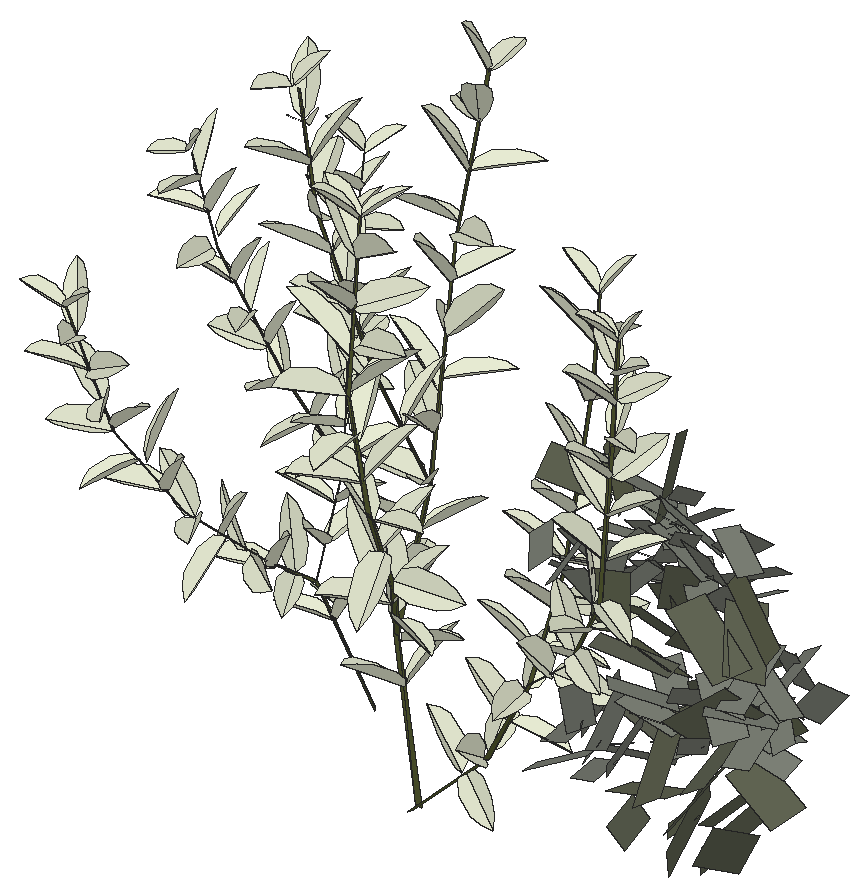
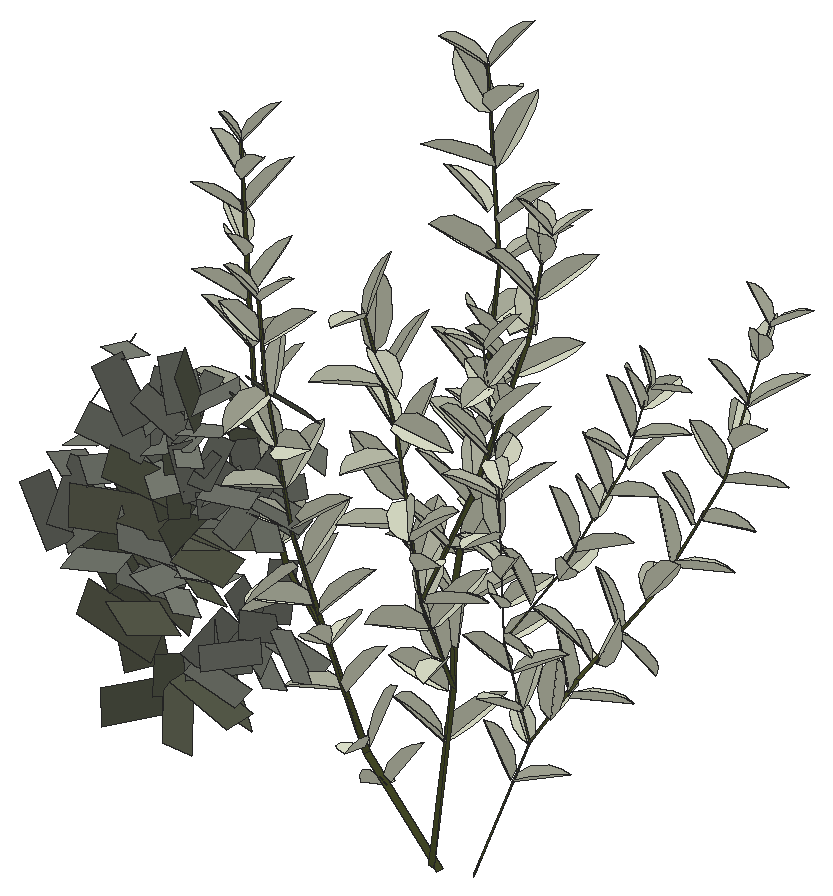
# SketchUp Ruby script. Lengths in inches.
U = 1.inch
M = Sketchup.active_model
def pt(a) = Geom::Point3d.new(a.map { |v| v * U })
def face(e, loops, mat)
  f = e.add_face(loops[0].map { |a| pt(a) })
  loops[1..].each { |l| e.add_face(l.map { |a| pt(a) }).erase! }
  f.material = f.back_material = mat if mat
  f
end
# faces: each face lists its corners as indices into pts; further lists are holes
def faces(e, pts, list, mat = nil) = list.each { |f| face(e, (f[0].is_a?(Array) ? f : [f]).map { |l| l.map { |i| pts[i] } }, mat) }
# xy, xz, yz: faces in a plane at the given z, y or x. An outline is a flat list of corners, or four numbers for a rectangle; further outlines are holes
def ring(l) = l.size == 4 ? [[l[0], l[1]], [l[2], l[1]], [l[2], l[3]], [l[0], l[3]]] : l.each_slice(2).to_a
def flat(e, list, mat, &to3) = list.each { |f| face(e, (f[0].is_a?(Array) ? f : [f]).map { |l| ring(l).map { |u, v| to3.(u, v) } }, mat) }
def xy(e, z, list, mat = nil) = flat(e, list, mat) { |x, y| [x, y, z] }
def xz(e, y, list, mat = nil) = flat(e, list, mat) { |x, z| [x, y, z] }
def yz(e, x, list, mat = nil) = flat(e, list, mat) { |y, z| [x, y, z] }
def lines(e, pts, list) = list.each { |a, b| e.add_line(pt(pts[a]), pt(pts[b])) }
# prism: a flat outline (further loops are holes) pulled along v
def prism(e, loops, v, mat = nil)
  f = face(e, loops, mat); d = Geom::Vector3d.new(v.map { |x| x * U })
  f.pushpull(f.normal.samedirection?(d) ? d.length : -d.length)
end
def box(e, o, s, mat = nil) = prism(e, [[o, [o[0] + s[0], o[1], o[2]], [o[0] + s[0], o[1] + s[1], o[2]], [o[0], o[1] + s[1], o[2]]]], [0, 0, s[2]], mat)
def at(x, y, z, deg = 0) = Geom::Transformation.translation(pt([x, y, z])) * Geom::Transformation.rotation(ORIGIN, Z_AXIS, deg.degrees)
def axes(o, x, y, z) = Geom::Transformation.new([*x, 0, *y, 0, *z, 0, *pt(o).to_a, 1])
def part(name) = M.definitions.add(name)
# library, detail: a bought-in or finely detailed component or shape, given as its bounding box
def library(name, o, s) = part(name).tap { |d| box(d.entities, o, s) }
def detail(e, o, s) = box(e.add_group.entities, o, s)
def put(e, d, t, mat = nil) = e.add_instance(d, t).tap { |i| i.material = mat if mat }
def group(e, t, mat = nil) = e.add_group.tap { |g| g.transformation = t; g.material = mat if mat }.entities
root = M.entities
M.materials.add("0ad16as01f6asdLeafVar1sfd015as60f1as6").color = [231, 235, 211]
M.materials.add("asdfasdf0165f6asdLeafVar1sfd015as60f1as6").color = [231, 235, 211]
M.materials.add("dw_stemssadfasdfa0sdf1s01d6w1").color = [90, 97, 50]
M.materials.add("viburnumblaasdfas0df1w06d").color = [98, 102, 84]
M.materials.add("viburnumbladsadfasdfad0w122").color = [125, 129, 119]
c1 = part("vdw_leaf\#1")
p = [[0,0,0],[-2.77,1.61,2.32],[-4.3125,6.1,4.5],[-3.97,13.49,6.09],[-2.47,18.57,6.3],[-0.2,22.73,5.75],
  [2.54,19.66,6.85],[4.3,15.93,7.09],[5.03,7.6,5.43],[3.32,1.76,2.74]]
faces(c1.entities,p,[[0,1,2,3,4,5],[0,5,6,7,8,9]],"0ad16as01f6asdLeafVar1sfd015as60f1as6")
c2 = part("dw_branch_3\#2")
p = [[-10.06,-1.6,62.9],[-0.2,1.54,-0.01],[-10.43,1.54,62.72],[0.18,-1.6,0.17],[-23.75,-21.66,88.91],[-25.7,-20.3,89.55],
  [13.4,11.62,104.56],[13.33,13.52,104.47],[-49.25,-41.87,130.3125],[-50.33,-40.21,130.71],[-4.97,21.13,143.98],[35.61,27.99,178.64],
  [-5.09,23.64,143.96],[35.32,29.14,178.46],[-67.7,-55.38,181.06],[-68.34,-54.45,181.62],[-22.8125,33.9,200.59],[-22.94,35.79,200.41],
  [56.61,36.78,229.75],[56.29,38.09,229.57],[-70.63,-67.46,248.85],[-70.72,-66.33,249.5],[-25.05,43.32,240.75],[-24.98,44.26,240.57]]
faces(c2.entities,p,[[0,1,2],[0,3,1],[4,2,5],[4,0,2],[6,0,2],[6,2,7],[8,4,5],[8,5,9],
  [10,6,7],[11,6,7],[10,7,12],[11,7,13],[14,8,9],[14,9,15],[16,10,12],[16,12,17],
  [18,11,13],[18,13,19],[20,14,15],[20,15,21],[22,16,17],[22,17,23]],"dw_stemssadfasdfa0sdf1s01d6w1")
c3 = part("dw_branch3\#2")
put(c3.entities,c1,axes([-70.33,-63.58,233.32],[-1.00752,0.412,0.78596],[-0.24851,-1.22189,0.32195],[0.83141,0.09817,1.01433]))
put(c3.entities,c1,axes([-66.93,-54.91,182.82],[-0.84976,-0.98359,0.33619],[0.99572,-0.74889,0.32577],[-0.05223,0.46521,1.22907]))
put(c3.entities,c1,axes([-46.12,-39.49,126.35],[1.23843,0.5364,0.23552],[-0.56438,0.94474,0.81599],[0.15707,-0.83465,1.07498]))
put(c3.entities,c1,axes([13.0625,13.13,104.77],[-1.01271,0.69982,-0.26884],[-0.74268,-0.99813,0.19939],[-0.10222,0.31872,1.21473]))
put(c3.entities,c1,axes([-18.87,30.42,186.42],[0.36309,1.06515,-0.56675],[-1.14134,0.49515,0.19939],[0.39128,0.45593,1.10754]))
put(c3.entities,c1,axes([-3.2,4.15,75.77],[-1.04153,0.55414,0.44243],[-0.23365,-1.01045,0.71554],[0.6695,0.50943,0.93801]))
put(c3.entities,c1,axes([23.2,19.41,136.3],[-0.65687,-1.11295,-0.05714],[1.05857,-0.61429,-0.20411],[0.15163,-0.1536,1.24868]))
put(c3.entities,c1,axes([-25.57,35.48,201.32],[-0.64726,0.62827,0.87973],[-0.71635,-1.0172,0.19939],[0.80962,-0.39773,0.87973]))
put(c3.entities,c1,axes([-36.37,-32.14,110.35],[-0.80747,1.09962,0.12544],[-0.83333,-0.50188,-0.96467],[-0.72833,-0.64487,0.96467]))
put(c3.entities,c1,axes([-9.89,26.72,156.79],[0.45529,1.02969,0.56572],[-1.16919,0.33753,0.32662],[0.11537,-0.64297,1.07744]))
put(c3.entities,c1,axes([-26.57,46.1,241.0625],[0.00015,0.80921,0.22536],[-0.83985,0.00446,-0.01542],[-0.01605,-0.22532,0.80906]))
put(c3.entities,c1,axes([-9.2,-2.58,61.06],[-1.10001,-0.40312,0.39014],[0.40883,-1.1116,0.00411],[0.35732,0.13566,1.14763]))
put(c3.entities,c1,axes([-69.91,-63.11,233.93],[1.36249,-0.1432,0],[0.13201,1.25603,0.5309],[-0.05549,-0.52799,1.26295]))
put(c3.entities,c1,axes([32.2,25.46,166.13],[0.06878,-1.29051,-0.05714],[1.22165,0.07415,-0.20411],[0.2113,-0.04403,1.24868]))
put(c3.entities,c1,axes([-5.68,-0.66,44.43],[-0.48448,-1.12287,0.17078],[0.98138,-0.33653,0.57135],[-0.48308,0.36756,1.04626]))
put(c3.entities,c1,axes([43.45,32.81,198.64],[0.5408,1.19584,0.14106],[-0.94242,0.32409,0.86557],[0.74952,-0.45533,0.98656]))
put(c3.entities,c1,axes([12.52,14.14,104.98],[1.02694,0.54888,0.41092],[-0.53566,1.05407,-0.06927],[-0.38969,-0.12321,1.13846]))
put(c3.entities,c1,axes([44.55,32.375,198.73],[-0.65687,-1.11295,-0.05714],[1.05857,-0.61429,-0.20411],[0.15163,-0.1536,1.24868]))
put(c3.entities,c1,axes([-5.67,21.17,141.44],[-1.10726,0.43603,-0.32953],[-0.49537,-1.03435,0.29588],[-0.17521,0.40597,1.12589]))
put(c3.entities,c1,axes([55.69,37.84,229.48],[0.18984,0.96334,0.18958],[-0.71996,0.0053,0.69399],[0.66755,-0.26823,0.69457]))
put(c3.entities,c1,axes([-21.52,36.85,205.2],[0.72606,-0.98817,0.14519],[0.94364,0.7084,0.10251],[-0.16885,0.05176,1.19664]))
put(c3.entities,c1,axes([-68.51,-56.35,196.07],[1.16319,0.72381,0],[-0.66725,1.0723,0.5309],[0.28049,-0.45075,1.26295]))
put(c3.entities,c2,at(0.01,-0.09,-0.02),"dw_stemssadfasdfa0sdf1s01d6w1")
put(c3.entities,c1,axes([-2.49,5.18,75.91],[0.78614,-0.90346,-0.30078],[0.86953,0.79562,-0.11715],[0.28546,-0.14014,1.16705]))
put(c3.entities,c1,axes([-23.125,-16.22,82.25],[0.32175,1.32576,0.12544],[-1.33153,0.31835,0.05068],[0.01989,-0.13382,1.3633]))
put(c3.entities,c1,axes([-23.75,41.99,230.3],[0.85958,-0.87451,0.14519],[0.66531,0.75721,0.62192],[-0.54076,-0.36226,1.01955]))
put(c3.entities,c1,axes([27.07,22.48,149.34],[0.92952,-0.64745,-0.62467],[0.50188,1.074,-0.36637],[0.71693,0.02135,1.04468]))
put(c3.entities,c1,axes([17.66,16.25,119.93],[-0.91649,0.83891,-0.3601],[-0.87434,-0.77966,0.40896],[0.0492,0.54447,1.14321]))
put(c3.entities,c1,axes([-68.37,-54.54,181.63],[0.32047,1.28399,0.35434],[-1.33153,0.31835,0.05068],[-0.03484,-0.35624,1.32241]))
put(c3.entities,c1,axes([-28.98,-27.1,96.48],[-0.8814,-0.35966,-0.98523],[0.75246,-1.11336,-0.26672],[-0.73065,-0.71272,0.91382]))
put(c3.entities,c1,axes([-15.23,28.43,172.72],[-1.21149,0.11898,0.32517],[-0.09739,-1.25259,0.09551],[0.33228,0.0667,1.21356]))
put(c3.entities,c1,axes([-17.5625,31.23,186.85],[-0.49275,-1.12287,0.14519],[0.95014,-0.33653,0.62192],[-0.53717,0.36756,1.01955]))
put(c3.entities,c1,axes([26.7,21.22,149.39],[-1.00104,0.22334,0.83093],[0.36894,-1.0402,0.72406],[0.77731,0.78134,0.72643]))
put(c3.entities,c1,axes([-31.125,-24.87,97.38],[0.75482,-0.86936,0.69068],[-0.00159,0.80023,1.00899],[-1.08766,-0.58016,0.45842]))
put(c3.entities,c1,axes([-71.21,-66.73,248.67],[0.25207,0.96771,0],[-0.8921,0.23237,0.38752],[0.375,-0.09768,0.92186]))
put(c3.entities,c1,axes([-24.11,41.05,229.55],[-1.11612,0.51924,-0.26884],[-0.56394,-1.10897,0.19939],[-0.15444,0.29694,1.21473]))
put(c3.entities,c1,axes([6.75,8.37,91.63],[-0.33418,-1.12287,0.39014],[1.13558,-0.33653,0.00411],[0.10478,0.36756,1.14763]))
put(c3.entities,c1,axes([-26,45.89,241.63],[-0.26986,-0.70824,-0.32129],[0.56818,-0.39091,0.38449],[-0.49365,-0.09775,0.63011]))
put(c3.entities,c1,axes([3.74,17.32,124.35],[0.22441,1.22913,-0.16274],[-1.07812,0.11178,-0.64246],[-0.61228,0.25367,1.07162]))
put(c3.entities,c1,axes([-5.44,22.27,140.88],[1.2203,0.00475,0.31374],[-0.097,1.20386,0.35905],[-0.29841,-0.37189,1.1663]))
put(c3.entities,c1,axes([-13.79,29.35,173.31],[0.83169,-0.90108,0.14519],[0.68877,0.73594,0.62192],[-0.55187,-0.34509,1.01955]))
put(c3.entities,c1,axes([-16.92,-7.26,72.98],[1.30647,0.30378,-0.27886],[0.07026,0.74892,1.14503],[0.40633,-1.10623,0.69861]))
put(c3.entities,c1,axes([4.8,17.55,125.22],[-0.25598,-1.17842,0.26559],[1.01553,-0.08455,0.60363],[-0.56975,0.35087,1.00767]))
put(c3.entities,c1,axes([5.3125,8.35,91.45],[0.00638,1.22913,-0.27714],[-1.16413,0.11178,0.46895],[0.48205,0.25367,1.13617]))
put(c3.entities,c1,axes([38.12,30.57,183.07],[1.12534,0.26182,-0.63833],[-0.46674,1.18829,-0.33545],[0.5081,0.51169,1.10563]))
put(c3.entities,c1,axes([-70.41,-60.38,214.47],[-0.41425,1.30587,0],[-1.20383,-0.38188,0.5309],[0.50605,0.16053,1.26295]))
put(c3.entities,c1,axes([37.03,28.75,180.67],[-1.12533,0.00102,-0.63799],[-0.00113,-1.2408,0],[-0.62497,0.00057,1.10237]))
put(c3.entities,c1,axes([30.71,25.35,165.96],[-0.1364,1.29314,0.22715],[-1.08768,-0.23921,0.70862],[0.73536,-0.11394,1.09026]))
put(c3.entities,c1,axes([-38.05,-30.84,110.67],[-0.31533,-1.27379,-0.2839],[1.018,-0.40311,0.67794],[-0.74394,-0.05723,1.08307]))
put(c3.entities,c1,axes([50.11,34.45,213.36],[-1.05669,0.74401,-0.05714],[-0.616,-0.82138,0.69675],[0.37221,0.60904,1.04705]))
put(c3.entities,c1,axes([-65.32,-58.78,200.07],[-1.14597,-0.19668,-0.6713],[0.21784,-1.26924,0],[-0.64812,-0.11124,1.139]))
put(c3.entities,c1,axes([-53.2,-43.37,143.59],[-0.72817,-1.09167,-0.2839],[0.82127,-0.72411,0.67794],[-0.71934,0.19815,1.08307]))
put(c3.entities,c1,axes([-61.1,-50.25,163.67],[-0.52887,1.19686,-0.30066],[-1.10762,-0.57104,-0.32484],[-0.42634,0.12264,1.23812]))
put(c3.entities,c1,axes([-54.12,-42.96,142.67],[0.32175,1.32576,0.12544],[-1.33153,0.31835,0.05068],[0.01989,-0.13382,1.3633]))
put(c3.entities,c1,axes([22.03,20.08,132.3],[1.17066,0.5058,-0.34078],[-0.35758,1.16671,0.50333],[0.49407,-0.35407,1.17172]))
put(c3.entities,c1,axes([-8.59,26.04,158.21],[-0.49275,-1.12287,0.14519],[0.95014,-0.33653,0.62192],[-0.53717,0.36756,1.01955]))
put(c3.entities,c1,axes([49.92,34.03,213.7],[1.24742,-0.35176,0.25024],[0.42127,1.159,-0.4708],[-0.09426,0.52477,1.20753]))
put(c3.entities,c1,axes([-70.34,-67.02,249.05],[-0.57048,-0.79684,0],[0.73827,-0.52855,0.24329],[-0.20203,0.14464,0.92729]))
put(c3.entities,c1,axes([56.04,36.81,228.63],[0.33451,-0.90845,-0.15237],[0.87636,0.33365,-0.06538],[0.11487,-0.11636,0.94597]))
put(c3.entities,c1,axes([-69.93,-60.58,214.88],[-0.45293,-0.99272,-0.78227],[1.14635,-0.58199,0.07483],[-0.40282,-0.65636,1.06615]))
put(c3.entities,c1,axes([-16.77,-8.59,72.7],[-1.22785,0.11509,0.53076],[-0.24879,-1.22495,-0.30991],[0.46742,-0.38989,1.16587]))
put(c3.entities,c1,axes([18.29,17.18,119.24],[1.19981,-0.45946,0.3029],[0.40159,1.22775,0.27158],[-0.37626,-0.1547,1.25575]))
put(c3.entities,c1,axes([-6.73,-0.68,43.74],[0.05346,1.22913,-0.27201],[-1.22696,0.11178,0.26396],[0.28163,0.25367,1.20164]))
put(c3.entities,c1,axes([-58.57,-48.42,160.98],[0.43385,-1.23789,0.39533],[1.04879,0.57965,0.66404],[-0.76727,0.09236,1.13122]))
put(c3.entities,c1,axes([-23.4,38.49,215.38],[0.06762,1.22913,-0.26884],[-1.23909,0.11178,0.19939],[0.21835,0.25367,1.21473]))
put(c3.entities,c1,axes([-22.21,-16.62,83.17],[-0.72817,-1.09167,-0.2839],[0.82127,-0.72411,0.67794],[-0.71934,0.19815,1.08307]))
put(c3.entities,c1,axes([-45.7,-40.77,126.53],[-1.33715,-0.0713,-0.0976],[0.07167,-1.28508,-0.04314],[-0.09306,-0.0492,1.31098]))
put(c3.entities,c1,axes([-22.39,38.51,216.12],[-0.49275,-1.12287,0.14519],[0.95014,-0.33653,0.62192],[-0.53717,0.36756,1.01955]))
c4 = part("Component\#315")
p = [[0.25,0,0],[2.05,0.01,0.35],[1.81,4.2,1.66],[0,4.19,1.3125]]
faces(c4.entities,p,[[0,1,2,3]],"viburnumbladsadfasdfad0w122")
c5 = part("viburnumblad2")
put(c5.entities,c4,axes([-19.23,-4.49,-32.18],[83.35428,0,0],[0,79.38502,0],[0,0,83.35428]))
c6 = part("vdw_leaf\#2")
p = [[0,0,0],[-2.77,1.61,2.32],[-4.3125,6.1,4.5],[-3.97,13.49,6.09],[-2.47,18.57,6.3],[-0.2,22.73,5.75],
  [2.54,19.66,6.85],[4.3,15.93,7.09],[5.03,7.6,5.43],[3.32,1.76,2.74]]
faces(c6.entities,p,[[0,1,2,3,4,5],[0,5,6,7,8,9]],"asdfasdf0165f6asdLeafVar1sfd015as60f1as6")
c7 = part("dg_branch_1\#2")
p = [[46.12,1.57,35.62],[46,5.42,35.41],[0.14,1.79,0.05],[0.26,-2.0625,0.27],[74.05,2.99,75.8],[74.11,5.28,75.58],
  [103.46,0.47,94.74],[104.03,2.92,94.84],[81.14,16.92,120.46],[81.2,18.78,120.24],[130.47,-5.6875,130.27],[130.58,-3.66,129.85],
  [80.82,34.4375,191.22],[80.64,35.93,190.9],[148.49,-14.56,203.24],[148.9,-12.8125,203.11],[81.08,37.95,226.93],[81.4,39.1,227.03],
  [157.45,-18.19,250.77],[157.7,-17.01,250.41]]
faces(c7.entities,p,[[0,1,2,3],[4,0,1],[4,1,5],[6,4,5],[6,5,7],[8,4,5],[8,5,9],[10,6,7],
  [10,7,11],[12,8,9],[12,9,13],[14,10,11],[14,11,15],[16,12,13],[16,13,17],[18,14,15],
  [18,15,19]],"dw_stemssadfasdfa0sdf1s01d6w1")
c8 = part("vdw_branch1\#3")
put(c8.entities,c6,axes([120.69,-2.42,117.31],[1.12221,-0.24063,-0.65809],[0.19207,1.24776,-0.12871],[0.65778,0.01392,1.11658]))
put(c8.entities,c6,axes([81,38.9,226.05],[0.7888,-0.58155,0],[0.48308,0.65523,0.47],[-0.28484,-0.38635,0.83138]))
put(c8.entities,c6,axes([78.08,12.69,106.05],[-1.43826,-0.02353,-0.03177],[0.0088,-1.31777,0.57755],[-0.03854,0.57714,1.31741]))
put(c8.entities,c6,axes([130.18,-4.73,130.41],[-0.38031,-1.29044,-0.11242],[1.20662,-0.31032,-0.51987],[0.47109,-0.24694,1.24081]))
put(c8.entities,c6,axes([157.08,-17.89,249.93],[-0.91355,0.40674,0],[-0.37496,-0.84216,0.38752],[0.15762,0.35401,0.92186]))
put(c8.entities,c6,axes([90.64,3.03,86.49],[0.32514,-0.85045,-0.99675],[0.69523,0.98247,-0.61148],[1.11061,-0.36604,0.67459]))
put(c8.entities,c6,axes([80.15,28.42,160.95],[-0.16039,0.95636,-1.06292],[-1.41646,0.03966,0.24943],[0.19509,1.07422,0.93709]))
put(c8.entities,c6,axes([126.74,-5.45,129.22],[-0.59819,0.96152,-0.6841],[-0.85772,0.12575,0.92675],[0.75427,0.88089,0.57856]))
put(c8.entities,c6,axes([133.22,-6.12,150.66],[-0.93823,0.76985,0.59124],[-0.47726,-1.08188,0.65135],[0.84525,0.24366,1.02405]))
put(c8.entities,c6,axes([80.43,22.89,141.32],[-1.42571,-0.19312,0.01373],[0.18338,-1.31425,0.5561],[-0.0621,0.5528,1.32692]))
put(c8.entities,c6,axes([33.14,0.88,26.42],[-0.13338,1.31536,0.04876],[-1.04528,-0.13221,0.7073],[0.72315,0.03348,1.07497]))
put(c8.entities,c6,axes([152.63,-15.08,221.76],[-1.28188,0.41945,0.0579],[-0.3638,-1.18547,0.53367],[0.21665,0.49113,1.23869]))
put(c8.entities,c6,axes([80.05,28.28,160.33],[-0.46732,-1.26661,0.40679],[1.27397,-0.40257,0.21004],[-0.07408,0.44645,1.30501]))
put(c8.entities,c6,axes([153.95,-14.8,235.875],[0.39005,1.07743,0.20605],[-0.96443,0.25296,0.50293],[0.42961,-0.3464,0.99807]))
put(c8.entities,c6,axes([80.2,24.22,141.74],[1.33062,-0.46576,0.02628],[0.44746,1.2746,-0.06608],[-0.00197,0.0722,1.37936]))
put(c8.entities,c6,axes([145.48,-12.5,188.92],[-1.32952,0.16983,0.16138],[-0.09299,-1.2361,0.53471],[0.21503,0.51548,1.22904]))
put(c8.entities,c6,axes([139.64,-9.18,171.24],[0.05682,1.30088,0.23414],[-1.13176,-0.05343,0.57151],[0.58357,-0.22963,1.13417]))
put(c8.entities,c6,axes([70.95,4.35,71.98],[-1.1081,-0.41873,0.64752],[0.33675,-1.28259,-0.25313],[0.6937,-0.04625,1.15721]))
put(c8.entities,c6,axes([59.85,4.55,56.17],[-0.26797,1.24526,0.35754],[-0.9369,-0.41634,0.74783],[0.83377,-0.10389,0.98674]))
put(c8.entities,c6,axes([33.11,3.36,25.66],[-0.57817,-1.07968,-0.5679],[1.11554,-0.21356,-0.7297],[0.49375,-0.78178,0.98363]))
put(c8.entities,c7,at(-0.21,0.34,-0.17),"dw_stemssadfasdfa0sdf1s01d6w1")
put(c8.entities,c6,axes([80.91,19.01,122.53],[-0.84258,1.13222,-0.27981],[-1.15093,-0.75138,0.42537],[0.18861,0.47293,1.3457]))
put(c8.entities,c6,axes([119.8,-1.22,114.1],[-1.3235,-0.25012,0.09101],[0.25933,-1.31572,0.15537],[0.05991,0.1698,1.33794]))
put(c8.entities,c6,axes([46.29,5.1,38.04],[0.98937,0.73827,-0.47585],[-0.72359,1.03721,0.10473],[0.44068,0.18581,1.20453]))
put(c8.entities,c6,axes([81.1875,33.03,184.45],[1.33883,0.26986,0.35053],[-0.09581,1.22087,-0.57399],[-0.42216,0.53228,1.20262]))
put(c8.entities,c6,axes([80.16,36.28,206.98],[-0.83993,0.85737,-0.6234],[-1.05964,-0.65701,0.5241],[0.02941,0.81391,1.07976]))
put(c8.entities,c6,axes([154.86,-16.15,234.87],[0.02509,-1.15302,-0.28506],[1.1487,-0.04894,0.29908],[-0.30202,-0.28195,1.11384]))
put(c8.entities,c6,axes([108.77,-0.33,101.14],[-0.47691,-1.03266,-0.72709],[1.25395,-0.29455,-0.40416],[0.15052,-0.81814,1.06325]))
put(c8.entities,c6,axes([89.79,3.01,85.87],[-0.61344,0.75518,0.8965],[-0.17758,-1.01824,0.73622],[1.13385,0.22574,0.58569]))
put(c8.entities,c6,axes([81.56,20.31,123.29],[0.37259,-1.3435,0.21057],[1.29385,0.32364,-0.22445],[0.16906,0.25791,1.34638]))
put(c8.entities,c6,axes([46.45,1.82,36.74],[-0.77883,0.29892,1.0614],[0.19124,-1.24314,0.49044],[1.08598,0.43329,0.67484]))
put(c8.entities,c6,axes([71.37,4.02,72.32],[0.72905,0.81546,-0.74421],[-0.66805,0.98958,0.42988],[0.8391,0.14186,0.97745]))
put(c8.entities,c6,axes([136.59,-5.88,150.53],[0.85845,-0.99897,-0.12437],[0.96526,0.81273,0.13453],[-0.02572,-0.18182,1.28292]))
put(c8.entities,c6,axes([80.375,38.8,225.86],[-0.25178,0.96778,0],[-0.89216,-0.23211,0.38752],[0.37503,0.09757,0.92186]))
put(c8.entities,c6,axes([74.43,7.99,85.38],[-1.05703,0.91669,-0.33543],[-0.95806,-0.87958,0.61531],[0.18697,0.6754,1.25659]))
put(c8.entities,c6,axes([76.57,9.74,89.32],[0.63146,-1.21538,0.33508],[1.18148,0.49387,-0.43517],[0.26321,0.48577,1.26593]))
put(c8.entities,c6,axes([81.6875,36.97,207.4],[0.09422,-1.04424,0.38486],[1.01646,0.1939,0.27727],[-0.33299,0.33382,0.98727]))
put(c8.entities,c6,axes([157.29,-17.17,249.98],[0.50586,-0.50586,0],[0.38853,0.38853,0.41105],[-0.29684,-0.29684,0.56115]))
put(c8.entities,c6,axes([79.92,15.8,106.09],[1.03917,-0.29343,-0.90675],[-0.14587,1.22131,-0.5624],[0.92163,0.5191,0.88824]))
put(c8.entities,c6,axes([61.95,3.88,56.26],[0.41243,-1.28546,0],[1.17466,0.37688,-0.54831],[0.5221,0.16751,1.23363]))
put(c8.entities,c6,axes([151.99,-14.79,208.15],[-0.48571,-1.21723,-0.32393],[1.25386,-0.50033,0],[-0.12005,-0.30087,1.31056]))
put(c8.entities,c6,axes([108.44,0.62,102.22],[0.82183,0.96078,0.38967],[-0.62327,0.08618,1.10203],[0.79141,-0.88661,0.51693]))
put(c8.entities,c6,axes([145.6,-10.56,188.62],[1.03241,-0.02554,-0.82693],[0.3944,1.11584,0.45794],[0.70325,-0.61672,0.89706]))
put(c8.entities,c6,axes([78.59,32.3,183.89],[-1.12675,-0.42036,0.43987],[0.5899,-0.98149,0.57312],[0.14901,0.70693,1.05726]))
put(c8.entities,c6,axes([152.08,-13.42,223.37],[0.79993,-0.44251,-0.69938],[0.68456,0.82615,0.26026],[0.41048,-0.60953,0.85515]))
put(c8.entities,c6,axes([140.71,-8.74,170.55],[0.41903,-1.24177,-0.32393],[1.26224,0.33728,0.33986],[-0.23168,-0.40836,1.26573]))
put(c8.entities,c6,axes([149.25,-12.53,205.78],[1.24456,0.38285,0.23414],[-0.42999,1.04826,0.57151],[-0.02056,-0.62679,1.13417]))
c9 = part("Component\#314")
p = [[0.14,0,0],[2.58,0.05,0.25],[2.44,5.11,2.64],[0,5.05,2.39]]
faces(c9.entities,p,[[0,1,2,3]],"viburnumblaasdfas0df1w06d")
c10 = part("viburnumblad1\#2")
put(c10.entities,c9,axes([-37.25,6.23,19.31],[75.98784,0,0],[0,65.50676,0],[0,0,75.98784]))
put(root,c3,axes([1192.89,291.63,3.91],[0.11088,0.06382,0.04174],[-0.06957,0.11109,0.02262],[-0.01961,-0.03323,0.15579]))
put(root,c3,axes([1199.15,288.14,0.8],[0.05022,0.15549,0],[-0.15549,0.05022,0],[0,0,0.20106]))
put(root,c5,axes([1213.24,287.5,23.46],[0.00132,0.00974,-0.00592],[-0.01063,-0.00165,-0.00484],[-0.00451,0.00633,0.00719]))
put(root,c5,axes([1212,282.6,24.66],[0.00896,0.00518,0.00557],[-0.00512,0.01053,-0.00146],[-0.00544,-0.00118,0.00865]))
put(root,c8,axes([1198.79,287.77,0.51],[0.13835,-0.02464,0],[0.02464,0.13835,0],[0,0,0.17291]))
put(root,c5,axes([1212.97,284.9,11.875],[0.00484,0.0109,0.00393],[-0.00707,0.00614,-0.00813],[-0.00911,0.00107,0.00791]))
put(root,c10,axes([1215.43,285.93,29.1875],[0.00062,0.00927,0.00842],[-0.01215,0.00581,-0.0055],[-0.00687,-0.00679,0.00799]))
put(root,c5,axes([1213.39,286.79,22.14],[0.008,0.00859,-0.00017],[-0.00687,0.00594,-0.00742],[-0.00498,0.00541,0.0075]))
put(root,c5,axes([1214.66,285.97,21.98],[0.00165,0.00828,-0.00613],[-0.01063,-0.00165,-0.00484],[-0.00434,0.00735,0.00651]))
put(root,c5,axes([1214.8,284.63,11.73],[-0.00076,0.01192,-0.00361],[-0.00919,-0.00341,-0.00868],[-0.0089,0.00223,0.00792]))
put(root,c5,axes([1214.8125,287.11,22.93],[-0.00614,0.00518,-0.0082],[-0.00794,-0.00715,0.00088],[-0.00475,0.00709,0.00648]))
put(root,c5,axes([1214.37,288.45,23.62],[-0.01,-0.00241,-0.00568],[-0.00201,-0.00892,0.00667],[-0.00557,0.00722,0.00577]))
put(root,c5,axes([1212.65,288.33,22.4375],[0.01,0.00241,0.00568],[0.00061,0.01041,-0.00507],[-0.00589,0.00485,0.00722]))
put(root,c5,axes([1212.83,283.23,23.64],[0.00946,-0.00383,0.00571],[0.00246,0.01108,0.00318],[-0.00637,-0.00125,0.00808]))
put(root,c5,axes([1213.04,286.46,11.62],[0.00591,-0.00596,0.00904],[0.00359,0.01104,0.00474],[-0.01042,0.00047,0.00632]))
put(root,c5,axes([1215.66,290.36,24.35],[-0.00169,0.00975,-0.0041],[-0.01002,-0.00286,-0.00259],[-0.00334,0.00343,0.00858]))
put(root,c5,axes([1214.08,285.23,10.625],[0.0076,0.00349,0.00917],[-0.0018,0.01107,-0.00252],[-0.00973,0.00035,0.00724]))
put(root,c5,axes([1214,286.64,12.84],[-0.00484,-0.0109,-0.00393],[0.00466,-0.0057,0.0098],[-0.01055,0.00253,0.0057]))
put(root,c10,axes([1215.91,287.42,27.46],[0.00699,0.00088,0.01038],[-0.00621,0.01278,0.0031],[-0.00893,-0.00592,0.00652]))
put(root,c5,axes([1216.04,290.73,12.28],[-0.00463,0.00496,-0.0092],[-0.00796,-0.0082,-0.00042],[-0.00678,0.00624,0.00678]))
put(root,c5,axes([1215.39,284.68,10.1],[0.00505,0.01138,0.0041],[-0.00637,0.00552,-0.00732],[-0.00911,0.00107,0.00791]))
put(root,c5,axes([1215.64,286.77,22.02],[-0.01044,-0.00252,-0.00593],[-0.00181,-0.00803,0.006],[-0.00557,0.00722,0.00577]))
put(root,c5,axes([1216.59,289.89,11.04],[0.00173,0.0098,-0.00563],[-0.00961,-0.00223,-0.00684],[-0.00663,0.00549,0.00752]))
put(root,c5,axes([1213.78,289.28,22.59],[-0.00132,-0.00974,0.00592],[0.00922,0.00313,0.00644],[-0.00695,0.00574,0.0058]))
put(root,c5,axes([1216.81,289.56,22.44],[-0.00122,0.00857,-0.00461],[-0.01002,-0.00286,-0.00259],[-0.0035,0.00446,0.00809]))
put(root,c5,axes([1214.87,288.24,22.1875],[-0.008,-0.00859,0.00017],[0.00566,-0.00462,0.00938],[-0.00647,0.00667,0.0055]))
put(root,c5,axes([1213.74,288.08,21.5],[0.00614,-0.00518,0.0082],[0.00724,0.00927,0.00063],[-0.0067,0.00499,0.00652]))
put(root,c5,axes([1216.96,290.44,23.48],[-0.00794,0.00459,-0.00546],[-0.00557,-0.00804,0.00123],[-0.00382,0.00415,0.0081]))
put(root,c5,axes([1214.73,286.77,11.2],[0.00076,-0.01192,0.00361],[0.0064,0.00373,0.01004],[-0.01075,0.00137,0.00569]))
put(root,c5,axes([1216.52,291.4,24.43],[-0.00954,-0.00326,-0.00362],[0.00113,-0.0093,0.00507],[-0.00471,0.00422,0.00764]))
put(root,c5,axes([1215.33,286.02,9.88],[0.00644,-0.0055,0.00764],[0.00359,0.01104,0.00474],[-0.00972,-0.00018,0.00726]))
put(root,c5,axes([1218.03,289.74,10.44],[-0.00445,0.00477,-0.00883],[-0.0086,-0.00885,-0.00045],[-0.00678,0.00624,0.00678]))
put(root,c5,axes([1217.41,290.86,11.28],[-0.00828,-0.00278,-0.00738],[-0.00265,-0.00909,0.0064],[-0.00743,0.00635,0.00594]))
put(root,c5,axes([1214.97,287.5,20.95],[-0.00127,-0.00935,0.00568],[0.00996,0.00338,0.00695],[-0.00695,0.00574,0.0058]))
put(root,c10,axes([1219.13,287.93,8.24],[0.0024,0.01209,-0.00232],[-0.01101,0.00036,-0.0095],[-0.00784,0.00332,0.00921]))
put(root,c5,axes([1218.25,288.61,27.1875],[0.00073,0.01102,-0.00295],[-0.01141,0.00071,-0.00016],[0.00003,0.00295,0.01104]))
put(root,c10,axes([1217.19,285.73,20.08],[-0.01129,-0.00613,-0.00067],[0.00417,-0.00777,0.01127],[-0.0047,0.00912,0.00614]))
put(root,c5,axes([1218.7,289.1,28.625],[-0.00749,0.00804,-0.00315],[-0.00863,-0.00712,0.00235],[-0.00031,0.00392,0.01074]))
put(root,c5,axes([1217.54,290.46,22.41],[-0.00996,-0.0034,-0.00378],[0.00101,-0.00837,0.00457],[-0.00471,0.00422,0.00764]))
put(root,c10,axes([1219.55,287.45,17.45],[0.00188,0.00994,-0.00772],[-0.0143,-0.00023,-0.00375],[-0.00243,0.00751,0.00854]))
put(root,c10,axes([1219.89,287,17.47],[-0.00372,0.0118,-0.00306],[-0.01362,-0.00502,-0.00283],[-0.00309,0.00191,0.01102]))
put(root,c10,axes([1219.18,283.97,6.59],[0.00499,0.00892,0.00903],[-0.00667,0.01209,-0.00778],[-0.01141,-0.0013,0.00685]))
put(root,c5,axes([1218,288.61,25.68],[0.00819,0.00724,-0.00098],[-0.00821,0.00902,-0.00193],[-0.00044,0.00202,0.01125]))
put(root,c5,axes([1216.67,291.55,22.97],[-0.00555,-0.00919,0.00035],[0.0077,-0.00439,0.00674],[-0.00547,0.00359,0.00747]))
put(root,c10,axes([1217.56,289.45,26.51],[0.00608,-0.01136,0.00423],[0.00607,0.0078,0.01224],[-0.01094,-0.0031,0.0074]))
put(root,c10,axes([1220.125,289.67,18.4],[-0.00938,0.00386,-0.00599],[-0.00819,-0.00718,0.008],[-0.00057,0.00892,0.00623]))
put(root,c10,axes([1219.79,288.71,19.22],[-0.0112,0.0013,-0.00343],[-0.00292,-0.0124,0.00476],[-0.00244,0.00473,0.0094]))
put(root,c10,axes([1219.84,287.34,6.09],[0.00721,0.00805,0.00636],[-0.00379,0.01064,-0.00917],[-0.00973,0.00288,0.00737]))
put(root,c5,axes([1219.48,289.41,27.11],[-0.01133,0.00035,-0.0015],[-0.0009,-0.01068,0.0043],[-0.00126,0.00434,0.0105]))
put(root,c5,axes([1219.45,286.55,15.99],[0.00933,0.00906,0.00093],[-0.00886,0.00934,-0.00204],[-0.00208,0.00083,0.01284]))
put(root,c5,axes([1220.73,285.87,14.6875],[0.00055,0.01289,-0.00188],[-0.01292,0.00032,-0.00165],[-0.00158,0.00193,0.01279]))
put(root,c5,axes([1221.01,286.26,16.42],[-0.00854,0.00917,-0.00359],[-0.00964,-0.00875,0.0006],[-0.00199,0.00305,0.01252]))
put(root,c10,axes([1218.62,290.18,20.15],[-0.00897,-0.00759,0.00065],[0.00732,-0.00776,0.00825],[-0.00418,0.00599,0.00812]))
put(root,c5,axes([1221.58,288.08,24.96],[-0.00115,0.01298,-0.0064],[-0.01441,0.00008,0.00199],[0.00223,0.00688,0.01234]))
put(root,c5,axes([1219.04,290.47,28.29],[-0.00853,-0.00755,0.00102],[0.00727,-0.00761,0.00446],[-0.00226,0.00398,0.01048]))
put(root,c5,axes([1220.63,286.04,12.96],[0.00895,0.00869,0.00089],[-0.00957,0.01008,-0.0022],[-0.00208,0.00083,0.01284]))
put(root,c5,axes([1220.91,287.62,23.23],[0.00912,0.00933,-0.00467],[-0.01186,0.01016,-0.00285],[0.00181,0.00573,0.01291]))
put(root,c5,axes([1218.43,290.54,26.64],[-0.00073,-0.01102,0.00295],[0.01017,0.00002,0.00259],[-0.00273,0.00304,0.01068]))
put(root,c5,axes([1219.39,289.85,25.64],[-0.00757,-0.0073,-0.00011],[0.00727,-0.00761,0.00446],[-0.00317,0.00314,0.01053]))
put(root,c5,axes([1222.41,289.14,26.45],[-0.01112,0.00864,-0.0042],[-0.00937,-0.00881,0.00635],[0.00161,0.00797,0.01181]))
put(root,c10,axes([1220.5625,282.93,10.22],[0.01357,-0.0015,0.0077],[-0.00069,0.01762,0.00453],[-0.00774,-0.0037,0.01228]))
put(root,c5,axes([1219.86,286.98,14.27],[0.01264,-0.00008,0.0032],[0.00017,0.01368,-0.00036],[-0.00319,0.00037,0.01263]))
put(root,c10,axes([1221.28,285.16,4.89],[0.00484,-0.00571,0.01239],[0.00394,0.01587,0.00555],[-0.01361,0.00143,0.00513]))
put(root,c5,axes([1222.07,286.84,14.87],[-0.01264,0.00008,-0.0032],[-0.00094,-0.01268,0.00342],[-0.00306,0.00351,0.01217]))
put(root,c10,axes([1219.0625,289.32,20.56],[0.00379,-0.01036,0.00596],[0.01309,0.006,0.00209],[-0.00395,0.00482,0.01088]))
put(root,c5,axes([1219.79,288.15,15.82],[0.00854,-0.00917,0.00359],[0.00887,0.00923,0.00245],[-0.00426,0.00084,0.01229]))
put(root,c10,axes([1221.13,286.76,9.59],[0.01227,-0.00323,0.0066],[0.00379,0.01612,0.00085],[-0.00658,0.00088,0.01266]))
put(root,c5,axes([1221.35,287.86,16.26],[-0.00933,-0.00906,-0.00093],[0.0081,-0.00886,0.00508],[-0.00417,0.00306,0.01196]))
put(root,c10,axes([1220.76,288.45,18.54],[-0.00969,-0.0086,0.00402],[0.01095,-0.00941,0.00625],[-0.00101,0.00665,0.01178]))
put(root,c10,axes([1221.8,287.56,4.14],[0.00403,-0.00389,0.01235],[0.00756,0.01368,0.00184],[-0.01119,0.00546,0.00538]))
put(root,c5,axes([1223,289.14,24.42],[-0.01458,-0.00076,0.00047],[0.00121,-0.01217,0.00796],[0.00032,0.00837,0.01162]))
put(root,c5,axes([1220.88,288.13,14.33],[-0.00055,-0.01289,0.00188],[0.01116,0.00015,0.00431],[-0.00466,0.00195,0.01201]))
put(root,c5,axes([1220.82,287.68,12.8],[0.00892,-0.00957,0.00375],[0.00799,0.0083,0.0022],[-0.00426,0.00084,0.01229]))
put(root,c5,axes([1222.14,287.52,13.26],[-0.00812,-0.00859,-0.00204],[0.0081,-0.00886,0.00508],[-0.00515,0.00206,0.01179]))
put(root,c5,axes([1220.92,289.3,22.46],[0.01161,-0.00902,0.00438],[0.00853,0.00943,-0.00297],[-0.0007,0.0056,0.01299]))
put(root,c10,axes([1221.83,284.6,8.33],[0.00765,-0.01303,0.00422],[0.01267,0.01016,0.00822],[-0.00817,-0.00039,0.01254]))
put(root,c5,axes([1221.43,290.34,23.79],[0.00115,-0.01298,0.0064],[0.01333,0.00146,0.00097],[-0.00132,0.00669,0.01246]))
put(root,c5,axes([1222.49,289.26,22.59],[-0.0086,-0.00967,0.00326],[0.01109,-0.00774,0.00569],[-0.00192,0.00675,0.01234]))
put(root,c5,axes([1222.58,290.77,25.64],[-0.0095,-0.00972,0.00486],[0.01109,-0.00774,0.00569],[-0.0009,0.00784,0.01189]))
put(root,c10,axes([1220.96,287.11,16.76],[0.00743,-0.01098,0.00888],[0.01612,0.00899,-0.00172],[-0.00302,0.0089,0.01251]))
put(root,c10,axes([1222.46,287.55,7.43],[0.00413,-0.01232,0.00597],[0.01417,0.00711,0.00487],[-0.00618,0.00389,0.01229]))
put(root,c10,axes([1227.16,282.63,21.32],[0.00623,0.01349,0.00121],[-0.0157,0.00724,0.00014],[-0.00044,-0.00098,0.01352]))
put(root,c10,axes([1222.73,285.55,14.24],[-0.01012,-0.01025,0.00891],[0.01634,-0.00922,0.0075],[0.00063,0.01164,0.0125]))
put(root,c5,axes([1227.41,289.23,15.09],[-0.00039,0.0109,-0.00675],[-0.01442,-0.00054,-0.00004],[-0.00029,0.00703,0.01137]))
put(root,c5,axes([1226.91,284.78,28.46],[0.00564,0.00974,-0.00221],[-0.01091,0.00622,-0.00021],[0.00111,0.00263,0.01119]))
put(root,c5,axes([1227.84,290.21,16.52],[-0.00964,0.00707,-0.00598],[-0.00922,-0.00808,0.00531],[-0.0008,0.00796,0.01071]))
put(root,c10,axes([1224.7,286.9,5.28],[-0.01097,-0.01069,0.00215],[0.01213,-0.01096,0.00739],[-0.00308,0.00597,0.01392]))
put(root,c5,axes([1226.8,282.3125,17.71],[0.01077,0.01069,0.00135],[-0.01074,0.01048,0.00267],[0.00094,-0.00284,0.01494]))
put(root,c10,axes([1223.98,289.2,12.6875],[-0.01045,-0.00476,0.01095],[0.01292,-0.01059,0.00773],[0.00429,0.01208,0.00936]))
put(root,c5,axes([1227.99,285.11,19.69],[0.00259,0.01229,-0.00001],[-0.01185,0.00249,-0.00335],[-0.00327,0.0007,0.01211]))
put(root,c10,axes([1227.24,283.25,21.54],[0.00918,0.0099,-0.00625],[-0.01245,0.01197,0.0007],[0.0045,0.00408,0.01216]))
put(root,c5,axes([1227.98,291.66,17.66],[-0.01322,-0.00136,-0.00142],[0.00017,-0.01043,0.00835],[-0.00196,0.00824,0.01034]))
put(root,c5,axes([1229.44,285.24,18.52],[-0.0062,0.01038,-0.0034],[-0.01088,-0.00717,-0.00204],[-0.00346,0.00185,0.01194]))
put(root,c5,axes([1226.35,283.23,19.74],[0.01523,-0.00004,0.00037],[-0.00005,0.01486,0.00338],[-0.00037,-0.00338,0.01485]))
put(root,c5,axes([1229.01,285.0625,16.75],[0.0027,0.01283,-0.00001],[-0.01066,0.00224,-0.00301],[-0.00327,0.0007,0.01211]))
put(root,c5,axes([1228.09,285.4,17.9375],[0.00987,0.007,0.00339],[-0.00618,0.00957,-0.0018],[-0.0039,-0.00027,0.01194]))
put(root,c5,axes([1226.76,283.27,15.91],[0.01462,-0.00004,0.00036],[-0.00005,0.01605,0.00365],[-0.00037,-0.00338,0.01485]))
put(root,c10,axes([1230.34,284.47,11.54],[0.00606,0.01155,0.00446],[-0.01316,0.00831,-0.00362],[-0.00493,-0.00229,0.01266]))
put(root,c10,axes([1229.57,284.18,22.99],[-0.00512,0.01258,-0.00225],[-0.01225,-0.00318,0.00944],[0.00707,0.00483,0.00942]))
put(root,c5,axes([1227.43,286.56,19.34],[0.01136,-0.00239,0.0048],[0.002,0.01232,0.0014],[-0.00498,-0.0005,0.01153]))
put(root,c5,axes([1228.05,291.68,15.65],[-0.00906,-0.00899,0.00397],[0.00943,-0.00624,0.00738],[-0.00308,0.00772,0.01046]))
put(root,c5,axes([1229.48,284.6875,16.87],[0.00856,0.00558,0.00422],[-0.00642,0.00891,0.00123],[-0.00278,-0.00341,0.01014]))
put(root,c5,axes([1230.61,284.38,15.64],[0.00178,0.0105,0.00298],[-0.0098,0.00211,-0.00159],[-0.00226,-0.0026,0.01051]))
put(root,c5,axes([1230.9,284.07,20.19],[0.00239,0.01136,-0.0048],[-0.01208,0.00314,0.00143],[0.00249,0.00434,0.01152]))
